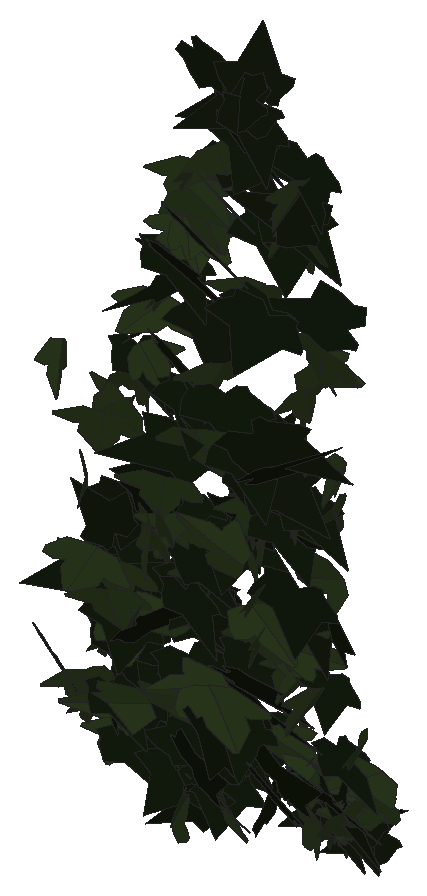
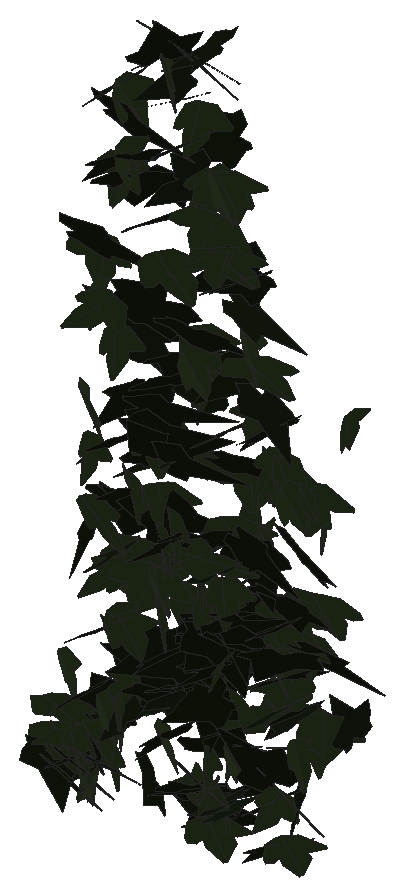
# SketchUp Ruby script. Lengths in millimetres.
U = 1.mm
M = Sketchup.active_model
def pt(a) = Geom::Point3d.new(a.map { |v| v * U })
def face(e, loops, mat)
  f = e.add_face(loops[0].map { |a| pt(a) })
  loops[1..].each { |l| e.add_face(l.map { |a| pt(a) }).erase! }
  f.material = f.back_material = mat if mat
  f
end
# faces: each face lists its corners as indices into pts; further lists are holes
def faces(e, pts, list, mat = nil) = list.each { |f| face(e, (f[0].is_a?(Array) ? f : [f]).map { |l| l.map { |i| pts[i] } }, mat) }
# xy, xz, yz: faces in a plane at the given z, y or x. An outline is a flat list of corners, or four numbers for a rectangle; further outlines are holes
def ring(l) = l.size == 4 ? [[l[0], l[1]], [l[2], l[1]], [l[2], l[3]], [l[0], l[3]]] : l.each_slice(2).to_a
def flat(e, list, mat, &to3) = list.each { |f| face(e, (f[0].is_a?(Array) ? f : [f]).map { |l| ring(l).map { |u, v| to3.(u, v) } }, mat) }
def xy(e, z, list, mat = nil) = flat(e, list, mat) { |x, y| [x, y, z] }
def xz(e, y, list, mat = nil) = flat(e, list, mat) { |x, z| [x, y, z] }
def yz(e, x, list, mat = nil) = flat(e, list, mat) { |y, z| [x, y, z] }
def lines(e, pts, list) = list.each { |a, b| e.add_line(pt(pts[a]), pt(pts[b])) }
# prism: a flat outline (further loops are holes) pulled along v
def prism(e, loops, v, mat = nil)
  f = face(e, loops, mat); d = Geom::Vector3d.new(v.map { |x| x * U })
  f.pushpull(f.normal.samedirection?(d) ? d.length : -d.length)
end
def box(e, o, s, mat = nil) = prism(e, [[o, [o[0] + s[0], o[1], o[2]], [o[0] + s[0], o[1] + s[1], o[2]], [o[0], o[1] + s[1], o[2]]]], [0, 0, s[2]], mat)
def at(x, y, z, deg = 0) = Geom::Transformation.translation(pt([x, y, z])) * Geom::Transformation.rotation(ORIGIN, Z_AXIS, deg.degrees)
def axes(o, x, y, z) = Geom::Transformation.new([*x, 0, *y, 0, *z, 0, *pt(o).to_a, 1])
def part(name) = M.definitions.add(name)
# library, detail: a bought-in or finely detailed component or shape, given as its bounding box
def library(name, o, s) = part(name).tap { |d| box(d.entities, o, s) }
def detail(e, o, s) = box(e.add_group.entities, o, s)
def put(e, d, t, mat = nil) = e.add_instance(d, t).tap { |i| i.material = mat if mat }
def group(e, t, mat = nil) = e.add_group.tap { |g| g.transformation = t; g.material = mat if mat }.entities
root = M.entities
M.materials.add("efeu1").color = [18, 25, 13]
M.materials.add("efeu2").color = [43, 57, 29]
c1 = part("ivyleaf_10")
p = [[0,12.8,-0.8],[-1.5,51.3,-10.9],[-4.9,51,-11.6],[-13.6,26.5,-7.3],[-13.2,15.9,-4.6],[-21.1,19.3,-7.2],
  [-29.5,16.3,-8.3],[-29.2,8.3,-6.2],[-19.7,-9.8,0.5],[-7.6,-13,4],[1,-12.2,5.8],[-0.4,51.1,-11.1],
  [-1.5,51.1,-10.9],[1,-12.4,5.9],[16.9,-12.4,3.5],[35.1,9.1,-5.1],[35,12.9,-6.1],[20.5,16.4,-4.9],
  [15.8,15,-3.8],[15.3,27.6,-7.1],[12.8,31.3,-7.8]]
faces(c1.entities,p,[[0,1,2,3,4,5,6,7,8,9,10],[11,12,0,13,14,15,16,17,18,19,20]],"efeu2")
c2 = part("ivyleaf_9")
p = [[39.1,54.8,31.7],[34.5,51.8,30.2],[-5.3,25.2,17.3],[-17.9,28.3,20.9],[-21.6,21.7,17],[-20.2,4.3,5.3],
  [-22.9,-0.3,2.5],[-17.1,-4,-0.6],[-2,-2.1,-1.2],[-0.7,-15.4,-10.1],[16.6,-22.3,-16.7],[21.1,-15.1,-12.5],
  [32.7,-10.7,-11],[46.1,-1.8,-6.6],[30.8,11.2,3.8]]
faces(c2.entities,p,[[0,1,2,3,4,5,6,7,8,9,10,11,12,13,14]],"efeu1")
put(root,c1,axes([1077.6,957,1774.6],[-0.11014,-0.83776,-0.20724],[-0.01883,0.20834,-0.83943],[1.64238,-0.05379,-0.02352]))
put(root,c2,axes([1054.3,883.8,1771.6],[0.21558,-0.51373,0.7615],[0.27708,-0.74753,-0.52596],[1.72615,0.18415,-0.01068]))
put(root,c2,axes([1103.4,908.8,1876.7],[-1.60044,0.11108,0.2626],[-0.49903,0.02004,-0.84811],[-0.21321,-0.88074,0.01382]))
put(root,c1,axes([1085.9,968,1651.8],[-0.94141,-0.60979,0.32314],[0.01475,-0.40246,-0.7476],[1.31336,-0.43258,0.24002]))
put(root,c2,axes([1090.9,931.6,1712.3],[0.59747,-0.12072,-0.80522],[-1.25036,0.47222,-0.32693],[0.91537,0.72383,0.079]))
put(root,c1,axes([1077.4,863.3,2163.1],[-0.00847,-0.85702,0.44016],[0.66042,-0.41205,-0.79878],[1.71057,0.15484,0.31057]))
put(root,c2,axes([1115,960.6,1722.1],[-1.40365,0.43604,-0.11187],[0.19046,-0.05055,-0.85675],[-0.83532,-0.74424,-0.00736]))
put(root,c1,axes([1102,876.5,1764.2],[-0.94627,-0.78401,-0.15345],[0.1624,0.12759,-0.92837],[1.51175,-0.50445,0.00368]))
put(root,c1,axes([1114.8,905.6,1885.1],[-1.50075,0.35253,0.19646],[-0.51322,-0.13942,-0.83218],[-0.57146,-0.8006,0.23143]))
put(root,c1,axes([1114.5,897.1,2075.7],[-1.58087,-0.4581,0.08244],[-0.13638,-0.04078,-0.94859],[0.87531,-0.83372,0.0011]))
put(root,c1,axes([1102.8,963.3,1703.9],[-0.49924,-0.5787,-0.57867],[0.45773,0.52633,-0.63537],[1.48877,-0.35588,0.0013]))
put(root,c1,axes([1129.8,906.1,2098.9],[-1.27836,0.30588,0.55125],[-1.08508,0.04902,-0.7219],[-0.51204,-0.86755,0.15357]))
put(root,c1,axes([1116.9,877.8,1743.7],[-0.19813,-0.85,-0.1351],[0.02969,0.1342,-0.85635],[1.63775,-0.10526,-0.00082]))
put(root,c2,axes([1095.4,963.6,1647],[0.10954,-0.77535,-0.3381],[0.22031,0.34291,-0.76668],[1.59469,0.00589,0.12914]))
put(root,c2,axes([1115.2,942,1955.2],[-1.48546,-0.1849,-0.40881],[0.77589,0.05031,-0.8011],[0.35661,-0.87965,0.04012]))
put(root,c1,axes([1116.3,869.1,1919.4],[1.73843,0.05819,-0.21679],[-0.41391,0.00472,-0.9151],[-0.10567,0.93879,0.01803]))
put(root,c1,axes([1116.9,927,2081.3],[-0.02622,-0.86903,0.30995],[0.09588,-0.31023,-0.86757],[1.75336,0.00397,0.05208]))
put(root,c2,axes([1101.2,928.9,1792.7],[0.29944,-0.84779,0.09383],[0.03639,-0.09188,-0.86227],[1.62296,0.15848,0.00202]))
put(root,c1,axes([1122.1,851.9,2029.6],[0.42573,-0.65508,-0.6532],[-0.03727,0.66852,-0.67715],[1.76024,0.17259,0.14364]))
put(root,c2,axes([1108.4,946.7,1884.8],[-0.53023,-0.68816,-0.48894],[0.40516,0.44096,-0.74194],[1.5547,-0.34961,0.0266]))
put(root,c2,axes([1108.5,962.9,1699.9],[0.05615,-0.859,-0.03641],[-0.00251,0.03639,-0.85951],[1.63632,0.02953,-0.00007]))
put(root,c2,axes([1132.2,956.5,1760.7],[-1.25251,-0.52279,0.2282],[0.02456,-0.36197,-0.79202],[1.08535,-0.59511,0.28127]))
put(root,c1,axes([1125.8,928.1,2126.7],[-0.67709,-0.63603,-0.57077],[0.47108,0.51507,-0.72823],[1.55673,-0.4325,-0.02789]))
put(root,c2,axes([1153.8,861.9,1967.4],[-0.20782,0.43978,0.84541],[-0.62122,0.7822,-0.44906],[-1.70395,-0.33881,0.06061]))
put(root,c1,axes([1130.9,885,1868.7],[-1.49949,-0.37149,-0.14448],[0.22617,0.08656,-0.87064],[0.7241,-0.79632,-0.02724]))
put(root,c2,axes([1143.9,954.8,1783.9],[-0.13318,-0.87274,-0.00572],[-0.01664,-0.00504,0.8755],[-1.66095,0.07003,-0.00831]))
put(root,c2,axes([1122.1,943,1914.3],[-0.32525,-0.84982,0.22084],[-0.06566,-0.21831,-0.86679],[1.66981,-0.17411,0.00893]))
put(root,c2,axes([1130.2,918.2,1833.2],[-0.57502,-0.8678,0.1042],[-0.08953,-0.09394,-0.9188],[1.66105,-0.30548,-0.01345]))
put(root,c1,axes([1144,885.7,1908.1],[-1.67458,-0.07199,0.1179],[-0.21894,-0.03898,-0.88233],[0.14555,-0.88689,0.02921]))
put(root,c1,axes([1127.8,910.2,1823.5],[0.94799,0.73589,0.03065],[0.03908,0.02311,-0.8886],[-1.40121,0.49851,-0.00405]))
put(root,c1,axes([1141.1,929.1,2121.4],[0.97915,-0.68339,-0.35174],[-0.02248,0.41618,-0.82588],[1.46263,0.46389,0.22277]))
put(root,c2,axes([1112.9,960.1,1726.3],[0.10822,-0.19691,0.83951],[1.11177,-0.61006,-0.18266],[1.20715,0.57951,0.09297]))
put(root,c2,axes([1157.9,921,2194.3],[-0.27248,0.92607,-0.02665],[0.00931,-0.02621,-0.93707],[-1.7632,-0.14325,-0.00083]))
put(root,c1,axes([1149.8,910,1849.9],[0.54344,-0.84895,0.02645],[0.0229,-0.02386,-0.89567],[1.61634,0.28577,0.0038]))
put(root,c2,axes([1178.7,932.4,2003.8],[-0.16669,0.01539,-0.90292],[-1.71276,-0.07679,0.08598],[-0.14267,0.9039,0.02268]))
put(root,c1,axes([1177.1,866.6,1759.3],[0.43263,0.11628,-0.94012],[-1.65307,-0.36025,-0.25458],[-0.7195,0.89762,0.01961]))
put(root,c2,axes([1141.2,924.1,2161.6],[0.21005,-0.8961,-0.23053],[-0.04262,0.2295,-0.90286],[1.76048,0.11247,0.00565]))
put(root,c2,axes([1145.2,873.7,1765.1],[0.21582,-0.78751,-0.35504],[-0.12836,0.34892,-0.79549],[1.63905,0.13102,-0.01555]))
put(root,c2,axes([1178.7,911.7,1984.5],[0.89047,0.25946,-0.72634],[-1.41595,-0.07221,-0.50504],[-0.38711,0.86097,0.17653]))
put(root,c1,axes([1174.8,916.9,2230.5],[1.42918,0.29794,-0.48827],[-0.87043,-0.17118,-0.80784],[-0.65378,0.87921,0.00817]))
put(root,c1,axes([1191.1,920.4,1845.6],[0.48923,0.28657,0.81958],[-1.2587,-0.48916,0.37847],[1.07061,-0.70606,0.07044]))
put(root,c1,axes([1166.5,904.8,2172.1],[0.51785,0.82406,0.33922],[-0.0986,0.3687,-0.85414],[-1.69316,0.23056,0.15349]))
put(root,c2,axes([1157.7,967.7,1675.7],[0.81843,-0.66202,-0.32096],[-0.00768,0.36964,-0.76783],[1.40021,0.38898,0.18339]))
put(root,c1,axes([1184.7,915,2260.5],[0.23166,-0.9228,-0.18496],[-0.01727,0.18535,-0.93067],[1.79112,0.12114,0.01495]))
put(root,c2,axes([1203.4,944.1,1879.1],[-0.5363,0.00115,0.84852],[-1.41576,-0.43046,-0.24646],[0.77689,-0.78365,0.13662]))
put(root,c1,axes([1201,873,1977.6],[-0.99982,0.48217,0.55768],[-0.89156,0.31044,-0.70968],[-1.0834,-0.70044,0.06936]))
put(root,c1,axes([1196,969.8,1639.1],[-1.08593,-0.57376,0.24648],[-0.15262,-0.26378,-0.79969],[1.17864,-0.56279,0.12354]))
put(root,c1,axes([1185.6,945.2,1727],[0.38168,-0.75179,0.37403],[0.2489,-0.35189,-0.77741],[1.57861,0.23725,0.03214]))
put(root,c2,axes([1198.8,944.9,1879.3],[0.56064,0.70969,-0.45704],[-0.33178,-0.42249,-0.76839],[-1.5719,0.34229,-0.00082]))
put(root,c2,axes([1204.4,944.2,1886],[0.81483,0.48634,-0.61673],[-0.7453,-0.47669,-0.64776],[-1.29576,0.58002,-0.01524]))
put(root,c1,axes([1189.7,948.6,1853.6],[-0.44137,0.83815,0.18605],[-0.05403,0.18512,-0.86937],[-1.63309,-0.23265,-0.02152]))
put(root,c1,axes([1198.9,939.9,1937.8],[-0.49582,-0.83736,-0.18676],[0.086,0.18152,-0.87689],[1.63055,-0.2642,-0.01054]))
put(root,c2,axes([1218.6,891,2283.9],[-1.25654,0.52595,-0.43888],[0.19443,-0.52712,-0.78539],[-1.28913,-0.59216,0.30932]))
put(root,c2,axes([1203.4,921.4,1658.7],[-0.74278,-0.69503,0.44921],[-0.39902,-0.39742,-0.79705],[1.52364,-0.44291,0.01026]))
put(root,c1,axes([1214.2,868.1,2004.7],[-0.90457,0.59938,0.49368],[-0.7545,0.31041,-0.75853],[-1.27076,-0.61096,0.09895]))
put(root,c2,axes([1231.8,898.3,2077.2],[-1.51149,-0.02153,0.46464],[-0.87323,-0.11469,-0.78956],[0.14536,-0.91294,0.08823]))
put(root,c2,axes([1195.7,855.9,1869.2],[-0.24535,0.48678,-0.84003],[-0.29851,0.82583,0.50262],[1.8235,0.20069,-0.03074]))
put(root,c2,axes([1185.5,955.1,1666.6],[0.49691,-0.8056,-0.07748],[0.02648,0.08587,-0.84593],[1.54006,0.25846,0.03954]))
put(root,c2,axes([1185.1,949.2,1846],[0.4772,-0.63994,-0.56159],[0.07596,0.59362,-0.65862],[1.61862,0.16081,0.19647]))
put(root,c1,axes([1194.9,868.7,1972.5],[0.39746,-0.70906,0.52201],[0.69229,-0.41909,-0.71479],[1.52606,0.37479,0.1883]))
put(root,c2,axes([1193.2,948.4,1868.6],[-0.63129,-0.45635,-0.68755],[0.82881,0.53262,-0.56362],[1.33405,-0.54686,0.02481]))
put(root,c1,axes([1219.3,941,1908.9],[-0.50484,-0.82491,0.24159],[-0.02623,-0.24871,-0.86438],[1.6357,-0.25858,0.0607]))
put(root,c1,axes([1217.2,947.4,1712.7],[0.16294,-0.75709,-0.40232],[0.13189,0.40911,-0.75512],[1.62637,0.04267,0.10154]))
put(root,c1,axes([1231.3,893.2,1985],[-1.2643,-0.56084,0.4009],[-0.45069,-0.33723,-0.86416],[1.23222,-0.69878,0.09527]))
put(root,c1,axes([1225,863,2050.1],[-1.57017,-0.39058,0.08448],[-0.12305,-0.06079,-0.9124],[0.75052,-0.8271,0.02716]))
put(root,c1,axes([1204.3,906.6,1747.2],[-1.46862,-0.25719,0.42322],[0.76606,0.13078,0.81339],[-0.54911,0.87033,0.00284]))
put(root,c1,axes([1248.5,936.1,1959.5],[0.13453,0.06033,0.90437],[-1.56694,-0.37508,0.08937],[0.72141,-0.82596,0.02547]))
put(root,c1,axes([1190.1,956.2,1650.1],[0.14128,-0.16001,0.86851],[1.54151,-0.33502,-0.13095],[0.66986,0.80472,0.11818]))
put(root,c2,axes([1225,939.2,1891.4],[-1.01779,-0.66799,0.26634],[-0.21883,-0.24822,-0.85341],[1.35104,-0.54343,0.06242]))
put(root,c1,axes([1219.8,936.8,1669.4],[-0.24943,0.81365,0.25695],[-0.18641,0.2439,-0.82228],[-1.61318,-0.15399,0.05529]))
put(root,c2,axes([1231,934.8,1629.8],[-0.33674,-0.13164,-0.83539],[0.34633,-0.83941,0.09373],[-1.57183,-0.15675,0.19962]))
put(root,c2,axes([1237.1,914,1701.2],[-1.53474,-0.36243,0.26858],[0.45714,0.12067,0.88403],[-0.72669,0.84134,-0.0111]))
put(root,c1,axes([1232.6,903.1,2348.8],[1.55395,0.23327,-0.45699],[-0.82276,-0.14982,-0.84887],[-0.52593,0.92361,-0.02228]))
put(root,c2,axes([1205.6,886.4,2199.7],[1.53686,-0.47226,-0.30843],[-0.42961,0.22304,-0.93249],[0.98381,0.83514,0.07462]))
put(root,c2,axes([1252.1,929.3,1663.4],[-0.20928,0.52151,0.69024],[-0.72996,0.59429,-0.51011],[-1.47581,-0.3679,0.15443]))
put(root,c2,axes([1209.1,923.7,2133],[0.36398,-0.89939,-0.15714],[0.1097,0.17213,-0.915],[1.73419,0.17788,0.09086]))
put(root,c2,axes([1212.3,895.7,2318.6],[0.04696,-0.95225,-0.1035],[0.1631,0.10532,-0.94851],[1.81569,0.01517,0.08788]))
put(root,c2,axes([1215.1,933.5,1951],[-0.13525,-0.77175,0.46903],[0.20737,-0.47437,-0.76402],[1.70622,-0.00352,0.13004]))
put(root,c2,axes([1202.3,943,1637.1],[0.57107,-0.58971,0.54178],[0.65518,-0.42738,-0.65585],[1.37606,0.44822,0.08743]))
put(root,c1,axes([1227,905.7,2349.2],[0.65206,0.90145,-0.01403],[-0.04568,-0.00589,-0.96415],[-1.71524,0.34285,0.02034]))
put(root,c2,axes([1206.7,875.2,2325.3],[1.77439,-0.34092,0.09087],[0.1418,-0.06071,-0.9922],[0.65635,0.93477,-0.0313]))
put(root,c1,axes([1243.8,891.4,2434.5],[-1.07668,-0.76176,0.26306],[-0.07796,-0.29381,-0.93889],[1.53182,-0.55038,0.13712]))
put(root,c1,axes([1236.9,936.1,1919.6],[0.47968,-0.79084,-0.33038],[0.14955,0.36424,-0.81194],[1.62431,0.20001,0.17232]))
put(root,c2,axes([1216.1,928.9,1783.8],[1.56925,-0.35959,-0.09504],[-0.16662,0.037,-0.89953],[0.68799,0.82916,-0.00108]))
put(root,c2,axes([1244.3,907,1766.3],[1.15699,0.03971,-0.70162],[-1.3331,0.1091,-0.60073],[0.10792,0.92192,0.10131]))
put(root,c1,axes([1244.2,895.7,2438.9],[0.1654,-0.97179,0.05974],[-0.00329,-0.06013,-0.97565],[1.85301,0.08663,-0.00707]))
put(root,c1,axes([1264.2,891.3,1800.5],[-0.21765,-0.10303,0.92284],[-0.85464,-0.80772,-0.14582],[1.54687,-0.46076,0.04928]))
put(root,c2,axes([1224.3,910.1,1814.1],[0.0342,-0.70626,-0.60136],[0.40091,0.58886,-0.68529],[1.71927,-0.12327,0.17176]))
put(root,c2,axes([1230.1,895.5,1903.4],[0.27017,-0.88574,-0.02827],[-0.0058,0.02814,-0.89704],[1.68658,0.14198,0.00144]))
put(root,c2,axes([1243.9,968.4,1667.7],[-0.77739,-0.71559,0.1997],[0.08283,-0.25055,-0.80878],[1.41152,-0.37941,0.15744]))
put(root,c2,axes([1246.1,937.4,1659.5],[-0.94443,-0.68415,-0.19503],[0.21789,0.1579,-0.84517],[1.3363,-0.50927,-0.00003]))
put(root,c1,axes([1261.6,841.5,1654.3],[0.02215,-0.02182,1.01459],[-0.90083,0.89742,0.02473],[-1.70847,-0.47347,0.00012]))
put(root,c2,axes([1240.8,935.8,1990.1],[-0.49088,-0.80843,-0.33464],[0.12924,0.32933,-0.84794],[1.66019,-0.26467,-0.03294]))
put(root,c1,axes([1249.8,897.7,2382.4],[-1.8109,0.00766,-0.18123],[0.34113,-0.10887,-0.94566],[-0.05299,-0.96247,0.10552]))
put(root,c2,axes([1240.6,888.5,1959.5],[0.699,-0.74157,-0.37263],[-0.15921,0.37233,-0.82343],[1.57146,0.36758,0.08232]))
put(root,c2,axes([1252.9,937.3,1958.2],[-0.43682,-0.81169,0.32932],[0.04443,-0.34598,-0.83649],[1.66652,-0.20353,0.10862]))
put(root,c2,axes([1263,915.4,2245.2],[-1.3664,-0.46742,-0.41007],[0.83034,0.06763,-0.84093],[0.84321,-0.82404,0.16358]))
put(root,c1,axes([1272.5,911.4,2197.4],[-0.03525,-0.91326,0.22885],[-0.00495,-0.22884,-0.91344],[1.79184,-0.0186,0.00198]))
put(root,c1,axes([1262.1,868.4,2419.4],[-0.98218,-0.69102,-0.53281],[0.75315,0.36636,-0.85844],[1.4801,-0.64498,0.08324]))
put(root,c2,axes([1309,925,2066.8],[-1.02095,0.14096,0.7455],[-1.38039,0.17269,-0.55456],[-0.4238,-0.90206,0.01034]))
put(root,c1,axes([1245.9,924.1,1643],[0.30981,-0.33966,0.83601],[1.48617,-0.37271,-0.30347],[0.86067,0.76583,0.22309]))
put(root,c1,axes([1275.2,959.2,1725.9],[0.63539,-0.79636,0.07531],[0.02418,-0.07631,-0.86333],[1.52221,0.33363,-0.01772]))
put(root,c2,axes([1270.6,868.1,2167.5],[-0.61444,-0.85758,0.21738],[0.01493,-0.23416,-0.91216],[1.68369,-0.31089,0.08742]))
put(root,c1,axes([1279.8,934.8,1999],[1.01039,-0.6513,-0.35879],[-0.0346,0.42936,-0.80628],[1.41477,0.47563,0.23652]))
put(root,c2,axes([1258.3,935.7,1980.4],[0.53859,-0.64597,-0.57979],[0.06658,0.61782,-0.67126],[1.65065,0.18585,0.21626]))
put(root,c1,axes([1279.6,875.8,2154.8],[0.35396,-0.8146,-0.43777],[0.22407,0.46376,-0.81294],[1.74571,0.10564,0.19311]))
put(root,c1,axes([1287.9,873.9,2207.9],[-0.63484,-0.93089,0.08302],[-0.04517,-0.07969,-0.98883],[1.77812,-0.33438,0.00452]))
put(root,c2,axes([1269.6,950.5,1728.8],[0.30876,-0.76049,-0.37401],[-0.15695,0.36483,-0.77759],[1.60527,0.18194,-0.00409]))
put(root,c2,axes([1315.5,924.7,2086.4],[-0.06861,0.03054,0.93121],[-1.64245,0.35017,-0.04489],[-0.66838,-0.86362,0.01472]))
put(root,c2,axes([1257.4,868.2,2140.4],[0.84776,-0.77207,0.27374],[0.3734,-0.20197,-0.8889],[1.51365,0.48224,0.06597]))
put(root,c1,axes([1288,946.3,1882.6],[0.61267,-0.77143,-0.31296],[-0.00584,0.33444,-0.82754],[1.58439,0.29954,0.11796]))
put(root,c2,axes([1278.4,911,1778.8],[-1.23365,-0.15584,-0.66212],[1.22237,0.16097,-0.66665],[0.42632,-0.91249,-0.00452]))
put(root,c2,axes([1267.7,866.8,2595.8],[1.00659,-0.81515,-0.27055],[-0.15162,0.26981,-0.96863],[1.62756,0.52928,0.07709]))
put(root,c2,axes([1275.5,944.3,1830.2],[0.29606,-0.81738,-0.29249],[-0.04478,0.29307,-0.83151],[1.65163,0.15446,0.02989]))
put(root,c1,axes([1300.9,930.4,2022.6],[-0.92142,-0.77953,0.06666],[0.044,-0.09261,-0.91509],[1.48836,-0.47985,0.06832]))
put(root,c1,axes([1296.7,935.4,1978.9],[0.91833,-0.75218,-0.18376],[0.03765,0.22842,-0.88306],[1.47317,0.46305,0.13712]))
put(root,c2,axes([1280.7,923.1,1769.1],[1.13047,-0.59289,-0.24997],[-0.36141,0.16351,-0.83906],[1.17002,0.62335,-0.01766]))
put(root,c1,axes([1296.5,836.2,2144.1],[-1.6109,-0.34341,-0.21699],[0.38756,0.07523,-0.9134],[0.66896,-0.87054,0.00667]))
put(root,c1,axes([1309.8,911.6,1942.7],[0.08742,0.07079,-0.93217],[-0.28255,0.922,0.0627],[1.75664,0.14478,0.05647]))
put(root,c2,axes([1282.6,877,2426],[1.58344,-0.46646,-0.20758],[-0.33492,0.11057,-0.95378],[0.91217,0.85034,0.01014]))
put(root,c2,axes([1336.2,918.9,2118.6],[-0.96916,-0.44858,-0.64625],[-0.78093,-0.50536,0.67411],[-1.27742,0.64928,0.0782]))
put(root,c2,axes([1267.3,934.3,1990],[0.64672,-0.18899,0.82754],[1.33291,-0.44124,-0.38835],[0.91282,0.7782,-0.01923]))
put(root,c1,axes([1302,856.9,2491.4],[-0.59949,-0.91313,-0.34822],[0.43719,0.28643,-0.9589],[1.80784,-0.37207,0.11642]))
put(root,c1,axes([1319.9,901.2,2306.8],[-0.99737,-0.70315,0.39512],[-0.45118,-0.31611,-0.87695],[1.46725,-0.57517,-0.00108]))
put(root,c2,axes([1305,926.9,1762],[-1.08545,-0.65308,-0.18702],[0.22769,0.14381,-0.86704],[1.27269,-0.58272,-0.00438]))
put(root,c2,axes([1313.9,925.6,1638.2],[0.07975,0.3968,0.84355],[0.26287,0.83244,-0.39844],[-1.75461,0.14275,-0.02135]))
put(root,c2,axes([1280.6,912.7,1810],[1.75614,-0.10296,0.15482],[0.29554,-0.00435,-0.92837],[0.19462,0.93562,0.01272]))
put(root,c1,axes([1318.1,923,2090.8],[-0.69978,-0.85905,0.01417],[-0.00733,-0.01377,-0.93443],[1.63515,-0.3677,0.00188]))
put(root,c2,axes([1288.9,833.2,1733.5],[0.00918,-0.12634,1.01915],[0.52161,-0.98204,-0.12303],[1.8836,0.27256,0.0291]))
put(root,c2,axes([1292.5,893.7,2471.6],[0.68648,-0.78077,-0.48096],[-0.05805,0.50633,-0.84482],[1.7443,0.32413,0.16117]))
put(root,c2,axes([1307.3,926.2,2072.4],[-0.70945,-0.23,0.8205],[1.32243,0.43637,0.438],[-0.93878,0.78851,-0.00306]))
put(root,c2,axes([1300.9,873.6,2179.3],[-0.40386,-0.8904,-0.37501],[0.25409,0.35324,-0.91426],[1.82114,-0.24674,0.0444]))
put(root,c2,axes([1307.5,886.9,1779.7],[-0.5515,-0.89135,-0.05788],[0.01892,0.05763,-0.93723],[1.69988,-0.28983,-0.00835]))
put(root,c2,axes([1295.7,901.5,2068.1],[1.18355,-0.53026,-0.4216],[-0.17916,0.49911,-0.7666],[1.27679,0.56157,0.28324]))
put(root,c2,axes([1308.4,944.2,1737.5],[-0.42172,-0.72927,0.4041],[0.09398,-0.42888,-0.7469],[1.584,-0.16871,0.1519]))
put(root,c1,axes([1350.6,822.5,2022.5],[0.49019,0.06853,1.0147],[-1.8937,0.23356,0.23679],[-0.40049,-1.02049,0.12234]))
put(root,c2,axes([1299.2,793.7,2433.3],[1.62491,-0.54645,-0.14226],[-0.19305,0.10527,-1.01312],[1.05719,0.85913,0.03365]))
put(root,c1,axes([1329.1,885,2558.8],[0.69298,-0.90729,-0.20859],[0.00085,0.22415,-0.97418],[1.7718,0.35475,0.08205]))
put(root,c1,axes([1330.3,892.4,1942],[0.32409,-0.88741,-0.064],[-0.01586,0.06357,-0.9036],[1.69324,0.17045,0.00378]))
put(root,c2,axes([1354.8,852,2574.7],[-1.54742,0.58648,0.01633],[-0.09333,-0.04012,-1.00064],[-1.11271,-0.81224,0.06122]))
put(root,c1,axes([1329.5,903.3,1886.8],[0.43205,-0.85457,0.14964],[0.11101,-0.1393,-0.88397],[1.64742,0.23351,0.02032]))
put(root,c2,axes([1297.6,917.6,1782.1],[0.85965,-0.54252,0.60462],[0.84246,-0.41569,-0.70368],[1.29634,0.62991,0.05636]))
put(root,c2,axes([1319.2,826.4,1788.4],[-0.07386,-0.66205,0.79895],[-0.08695,-0.79764,-0.66319],[1.97286,-0.05994,0.00068]))
put(root,c2,axes([1337.2,882.6,2567.1],[-0.98887,-0.43373,0.73756],[1.07234,0.47597,0.67681],[-1.22554,0.76643,-0.00292]))
put(root,c2,axes([1362.6,853.5,2572.2],[-1.84897,0.24702,-0.02149],[-0.06831,-0.22609,-0.97616],[-0.46694,-0.94507,0.22791]))
put(root,c1,axes([1343.9,942.5,1840.3],[-0.46589,-0.80969,0.25482],[-0.03021,-0.26079,-0.84391],[1.61523,-0.23842,0.05772]))
put(root,c1,axes([1339.6,958.9,1736.6],[0.46089,-0.78972,-0.26626],[0.07829,0.28826,-0.81756],[1.58419,0.21551,0.11786]))
put(root,c1,axes([1338.8,899.1,1888.2],[-1.68976,-0.31401,-0.19448],[0.33653,0.08319,-0.94155],[0.61718,-0.90509,-0.01906]))
put(root,c2,axes([1318.6,857.6,2535.4],[1.29449,-0.70973,-0.16453],[-0.24518,0.10438,-0.98281],[1.36473,0.69195,-0.0205]))
put(root,c1,axes([1322.4,826.3,1833],[1.7495,0.33945,0.34972],[0.62509,0.12013,-0.97991],[-0.6853,0.97615,-0.00102]))
put(root,c1,axes([1342.8,931.4,2025.9],[1.04383,-0.71148,-0.19551],[0.00567,0.24574,-0.88592],[1.40428,0.52787,0.14891]))
put(root,c2,axes([1341.4,884.8,2501.5],[-0.86434,-0.78601,0.39722],[-0.0514,-0.43428,-0.89024],[1.67532,-0.41885,0.17762]))
put(root,c2,axes([1337.8,931.8,2016],[-0.21606,-0.86843,-0.27563],[0.07885,0.27255,-0.8758],[1.73226,-0.12073,0.00549]))
put(root,c2,axes([1330.9,959.2,1724.4],[0.53913,-0.76236,0.28741],[0.17942,-0.27157,-0.81327],[1.5402,0.29849,-0.00587]))
put(root,c2,axes([1341.7,862.6,2131.6],[-0.30362,-0.94984,-0.18853],[0.04933,0.18681,-0.96313],[1.84234,-0.16154,-0.00528]))
put(root,c1,axes([1338.8,909.9,1756],[-1.04425,-0.4166,-0.6461],[1.06659,0.3266,-0.68652],[1.00153,-0.78219,0.05746]))
put(root,c1,axes([1334.7,888.9,1911.4],[1.46399,0.24532,0.51473],[0.91155,0.19104,-0.80681],[-0.58886,0.90563,0.03076]))
put(root,c1,axes([1362.9,933.5,1838.4],[-0.17154,-0.66178,0.58659],[0.04142,-0.59111,-0.66353],[1.68254,-0.05292,0.07614]))
put(root,c1,axes([1369.3,949.4,1728],[0.23353,-0.85447,0.00344],[-0.00486,-0.00384,-0.86323],[1.62623,0.12269,-0.00307]))
put(root,c2,axes([1352.6,855.9,2553.5],[-0.03334,-0.99155,0.12454],[-0.05315,-0.12402,-0.99138],[1.90121,-0.02086,-0.02553]))
put(root,c1,axes([1377.6,964.4,1696.3],[-0.53395,-0.73476,0.32647],[-0.06702,-0.33421,-0.78245],[1.52875,-0.27129,0.07972]))
put(root,c2,axes([1365.2,895.6,2402.8],[-0.8841,-0.82134,-0.2699],[0.20788,0.24819,-0.94325],[1.63224,-0.47649,-0.02606]))
put(root,c1,axes([1371.1,971,1644.2],[-0.74649,0.72193,-0.14794],[0.09236,-0.14192,-0.82123],[-1.39949,-0.39445,0.02471]))
put(root,c2,axes([1394.9,969.6,1667.8],[-1.59589,0.03192,0.0324],[-0.07526,-0.21612,-0.81051],[-0.04277,-0.81085,0.21731]))
put(root,c2,axes([1389.1,951.4,1672.3],[0.03543,0.1073,0.85761],[-0.11555,0.85586,-0.10577],[-1.64087,-0.05795,0.02596]))
put(root,c1,axes([1379,912.6,2194.6],[-0.36096,-0.88656,-0.28977],[0.21975,0.27111,-0.90504],[1.76149,-0.21549,0.05353]))
put(root,c2,axes([1354.3,876.6,1711.9],[0.19271,-0.4855,0.82162],[0.56305,-0.76957,-0.4912],[1.72684,0.3051,0.06847]))
put(root,c1,axes([1384.3,921,1655.3],[0.87467,-0.61766,-0.38922],[-0.18576,0.40381,-0.75606],[1.37699,0.44682,0.14524]))
put(root,c2,axes([1378.2,853.5,2320.8],[-0.69314,-0.79718,0.42304],[-0.19264,-0.41723,-0.87337],[1.70675,-0.37084,0.07323]))
put(root,c1,axes([1382.6,891.8,2423.4],[0.09566,-0.80906,0.56172],[0.15844,-0.55694,-0.80964],[1.86783,0.08868,0.03991]))
put(root,c1,axes([1379,919.3,1715.3],[-0.57564,-0.13498,0.86565],[0.53084,-0.88297,-0.04022],[1.58066,0.24738,0.32876]))
put(root,c1,axes([1387.9,889.9,2405.2],[-1.42438,0.61876,0.11802],[-0.1679,0.07851,-0.97107],[-1.18704,-0.75358,-0.00426]))
put(root,c1,axes([1404,927.1,1967.3],[0.88242,-0.35778,-0.75299],[-0.95589,0.56781,-0.57906],[1.26637,0.67791,0.0876]))
put(root,c1,axes([1389.3,960.8,1648],[0.17864,-0.83687,-0.10613],[-0.00826,0.1063,-0.84208],[1.60546,0.09367,0.00748]))
put(root,c1,axes([1387.5,960.5,1651.4],[0.64975,-0.7606,-0.15971],[0.08775,0.19396,-0.82512],[1.47654,0.32318,0.11932]))
put(root,c2,axes([1379.8,953.5,1825.1],[-0.36278,-0.82398,0.23187],[-0.03979,-0.23299,-0.84517],[1.62861,-0.18924,0.031]))
put(root,c2,axes([1374.1,865.4,2107],[0.07154,-0.57969,-0.79119],[-0.03982,0.79112,-0.58063],[1.86628,0.0391,0.01794]))
put(root,c2,axes([1370.5,961.5,1656.1],[0.49572,-0.80929,-0.00177],[0.04849,0.01006,-0.84974],[1.53949,0.26028,0.02733]))
put(root,c2,axes([1374.6,925.2,1913.3],[0.12768,-0.87143,0.19437],[0.01546,-0.19432,-0.87398],[1.69919,0.06725,-0.00665]))
put(root,c1,axes([1385,903.4,1878.4],[0.1661,0.41807,0.81576],[0.14238,0.81346,-0.4249],[-1.73874,0.10655,0.04313]))
put(root,c2,axes([1430.4,853.5,2447.3],[-1.04082,0.44439,0.689],[-0.98372,0.45602,-0.70439],[-1.21125,-0.75222,-0.01998]))
put(root,c2,axes([1375.5,892.8,2425.5],[0.15783,-0.86405,-0.46532],[0.17822,0.47181,-0.85942],[1.85924,0.02812,0.12188]))
put(root,c2,axes([1389.9,888.2,1963.4],[-1.43457,-0.12484,-0.60898],[1.12976,0.13963,-0.76337],[0.35127,-0.95892,-0.03188]))
put(root,c2,axes([1379.6,912.4,2060.1],[0.3006,-0.83646,-0.36525],[-0.03113,0.36803,-0.84989],[1.73683,0.15137,0.04799]))
put(root,c2,axes([1373.8,873.7,1728.7],[-0.06532,-0.10138,0.94975],[0.74881,-0.86749,-0.07838],[1.65645,0.38816,0.07289]))
put(root,c2,axes([1370.7,916.4,1710.3],[1.51783,-0.46356,0.2332],[0.38847,-0.11288,-0.92244],[0.90798,0.82321,0.00483]))
put(root,c1,axes([1406.1,906.4,2246.3],[-0.83856,0.77275,0.36419],[-0.34816,0.31492,-0.88954],[-1.58814,-0.47706,0.00271]))
put(root,c2,axes([1441.9,899.8,2303],[-1.14746,0.29819,0.70138],[-1.21777,0.2878,-0.67239],[-0.78801,-0.87898,0.01778]))
put(root,c2,axes([1424.3,969.8,1659.7],[-1.48102,0.29972,-0.02469],[0.02294,-0.03734,-0.83334],[-0.57189,-0.77767,0.0305]))
put(root,c1,axes([1405.8,926.3,2051.3],[-0.15901,-0.76376,-0.51858],[0.18144,0.51078,-0.76763],[1.74761,-0.12252,0.03251]))
put(root,c1,axes([1411.4,956.2,1671.5],[-0.6489,-0.74989,0.18335],[0.0679,-0.21553,-0.81515],[1.46766,-0.32158,0.11878]))
put(root,c2,axes([1392.5,953.2,1740.2],[0.42226,-0.78855,-0.28779],[-0.11795,0.28147,-0.81902],[1.59324,0.22983,0.01564]))
put(root,c1,axes([1411.6,857.2,2482.1],[0.00018,-0.97415,0.37068],[0.0767,-0.3704,-0.97342],[1.9822,0.01442,0.03763]))
put(root,c1,axes([1425.9,966.7,1680.8],[-1.38538,-0.2466,0.35468],[-0.62185,-0.14031,-0.76813],[0.5378,-0.79748,0.02547]))
put(root,c1,axes([1397.5,910.4,2232.2],[-0.62956,-0.43591,-0.78512],[0.92359,0.61723,-0.54715],[1.43805,-0.58725,0.0077]))
put(root,c2,axes([1395.9,966.6,1659.2],[0.10386,-0.81841,-0.20257],[0.0484,0.2045,-0.81935],[1.60386,0.04683,0.03785]))
put(root,c2,axes([1418.2,798.5,2351.5],[-1.68951,-0.23885,-0.3304],[0.62616,0.04785,-0.91855],[0.45824,-0.946,0.03696]))
put(root,c1,axes([1429.5,962.1,1716.7],[1.2747,0.03856,-0.54108],[-1.02984,-0.01301,-0.67073],[-0.07266,0.86092,0.0141]))
put(root,c1,axes([1416.4,922.3,2107.2],[0.87321,-0.81451,0.04054],[0.0509,-0.03146,-0.93481],[1.55126,0.45952,0.00785]))
put(root,c1,axes([1425,951.2,1672.4],[-0.9012,-0.62613,0.30879],[-0.13396,-0.32839,-0.77383],[1.32191,-0.46014,0.13209]))
put(root,c1,axes([1411.7,969.5,1686.5],[0.46776,0.81089,-0.02227],[-0.01189,-0.02138,-0.84732],[-1.54383,0.24585,-0.00022]))
put(root,c2,axes([1427.8,971.3,1655.7],[0.11221,0.84178,0.00722],[0.02801,0.0062,-0.84372],[-1.60189,0.05907,-0.01425]))
put(root,c2,axes([1404.3,884.5,2502.6],[0.04043,-0.98035,0.17877],[-0.06157,-0.17939,-0.97993],[1.89557,0.01508,-0.03564]))
put(root,c2,axes([1439.8,973.3,1643.6],[-1.45371,0.32911,0.01305],[-0.02408,0.00361,-0.83171],[-0.6264,-0.76393,0.0017]))
put(root,c2,axes([1395.6,813.1,2140.1],[0.76838,0.96973,-0.07118],[0.03403,0.06966,1.05037],[1.85025,-0.404,0.01024]))
put(root,c2,axes([1394.3,811.1,2191.1],[0.09486,-0.09772,-1.04658],[0.67984,0.98697,-0.07514],[1.88145,-0.35171,0.07992]))
put(root,c1,axes([1403.1,876.6,2168.2],[0.32186,-0.27585,0.91667],[1.11771,-0.70521,-0.32056],[1.43875,0.60956,0.04397]))
put(root,c2,axes([1401.6,945.9,1674.7],[0.6066,-0.76764,0.20371],[0.14452,-0.18904,-0.83117],[1.50461,0.32764,-0.00229]))
put(root,c2,axes([1425.1,901.4,1930.6],[0.84304,-0.25191,-0.78186],[-1.18789,0.47428,-0.50643],[1.01638,0.76326,0.05663]))
put(root,c1,axes([1428.9,861,1858.7],[-0.00465,-0.90618,0.38921],[0.02463,-0.3892,-0.90609],[1.87683,0.00286,0.01286]))
put(root,c1,axes([1425.9,921.4,1683.5],[-0.4351,-0.76632,-0.46253],[0.24797,0.44381,-0.7997],[1.6854,-0.26313,-0.00175]))
put(root,c1,axes([1430.6,944.3,1764.3],[0.26266,-0.84145,-0.17747],[-0.0783,0.17307,-0.8526],[1.6348,0.14348,-0.01232]))
put(root,c1,axes([1437.8,872,2279.2],[-1.69083,0.3289,0.27472],[-0.48384,0.10455,-0.94729],[-0.65658,-0.92402,-0.0094]))
